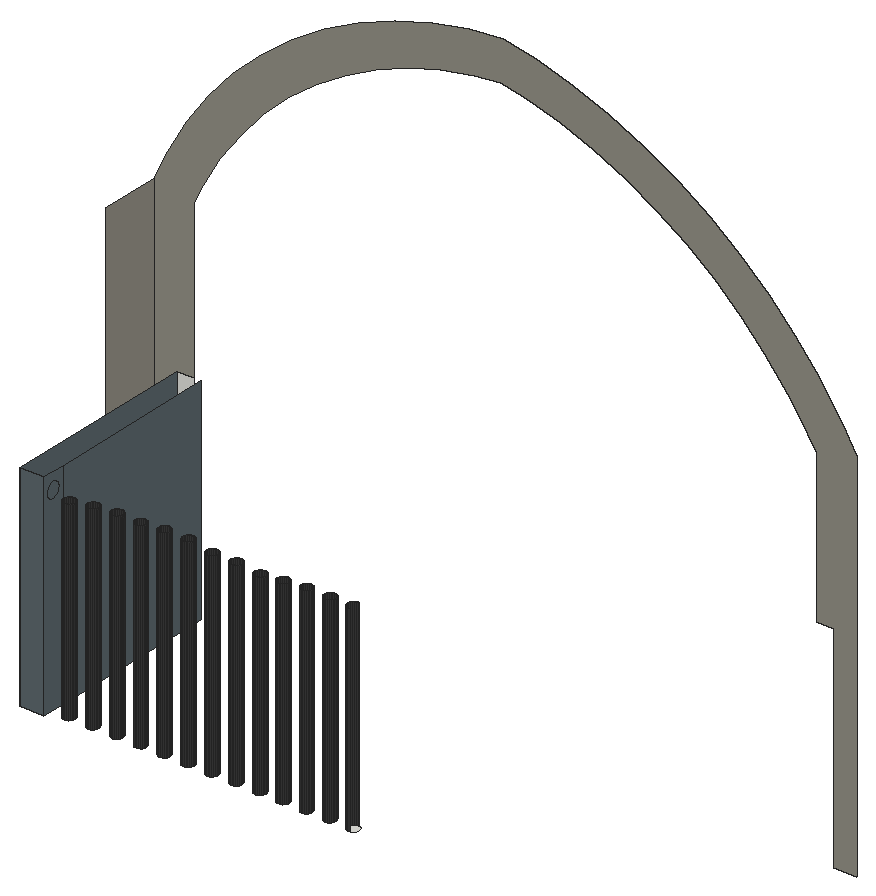
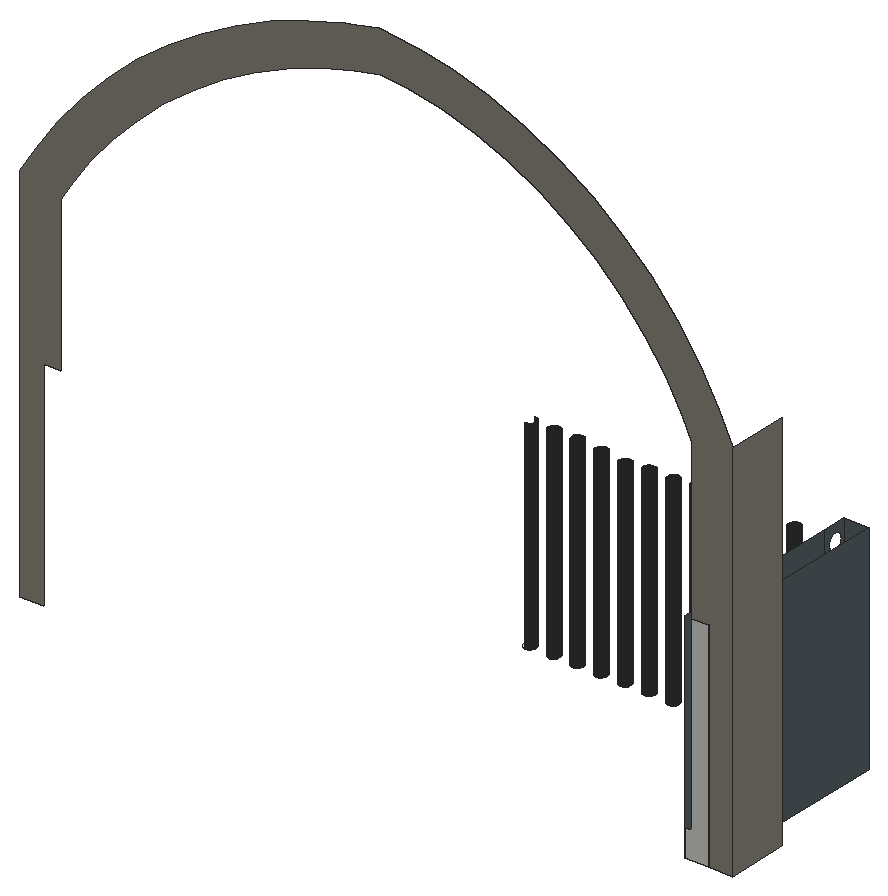
# SketchUp Ruby script. Lengths in inches.
U = 1.inch
M = Sketchup.active_model
def pt(a) = Geom::Point3d.new(a.map { |v| v * U })
def face(e, loops, mat)
  f = e.add_face(loops[0].map { |a| pt(a) })
  loops[1..].each { |l| e.add_face(l.map { |a| pt(a) }).erase! }
  f.material = f.back_material = mat if mat
  f
end
# faces: each face lists its corners as indices into pts; further lists are holes
def faces(e, pts, list, mat = nil) = list.each { |f| face(e, (f[0].is_a?(Array) ? f : [f]).map { |l| l.map { |i| pts[i] } }, mat) }
# xy, xz, yz: faces in a plane at the given z, y or x. An outline is a flat list of corners, or four numbers for a rectangle; further outlines are holes
def ring(l) = l.size == 4 ? [[l[0], l[1]], [l[2], l[1]], [l[2], l[3]], [l[0], l[3]]] : l.each_slice(2).to_a
def flat(e, list, mat, &to3) = list.each { |f| face(e, (f[0].is_a?(Array) ? f : [f]).map { |l| ring(l).map { |u, v| to3.(u, v) } }, mat) }
def xy(e, z, list, mat = nil) = flat(e, list, mat) { |x, y| [x, y, z] }
def xz(e, y, list, mat = nil) = flat(e, list, mat) { |x, z| [x, y, z] }
def yz(e, x, list, mat = nil) = flat(e, list, mat) { |y, z| [x, y, z] }
def lines(e, pts, list) = list.each { |a, b| e.add_line(pt(pts[a]), pt(pts[b])) }
# prism: a flat outline (further loops are holes) pulled along v
def prism(e, loops, v, mat = nil)
  f = face(e, loops, mat); d = Geom::Vector3d.new(v.map { |x| x * U })
  f.pushpull(f.normal.samedirection?(d) ? d.length : -d.length)
end
def box(e, o, s, mat = nil) = prism(e, [[o, [o[0] + s[0], o[1], o[2]], [o[0] + s[0], o[1] + s[1], o[2]], [o[0], o[1] + s[1], o[2]]]], [0, 0, s[2]], mat)
def at(x, y, z, deg = 0) = Geom::Transformation.translation(pt([x, y, z])) * Geom::Transformation.rotation(ORIGIN, Z_AXIS, deg.degrees)
def axes(o, x, y, z) = Geom::Transformation.new([*x, 0, *y, 0, *z, 0, *pt(o).to_a, 1])
def part(name) = M.definitions.add(name)
# library, detail: a bought-in or finely detailed component or shape, given as its bounding box
def library(name, o, s) = part(name).tap { |d| box(d.entities, o, s) }
def detail(e, o, s) = box(e.add_group.entities, o, s)
def put(e, d, t, mat = nil) = e.add_instance(d, t).tap { |i| i.material = mat if mat }
def group(e, t, mat = nil) = e.add_group.tap { |g| g.transformation = t; g.material = mat if mat }.entities
root = M.entities
M.materials.add("[Color M07]").color = [58, 58, 58]
M.materials.add("[Formica Graystone]").color = [149, 146, 135]
M.materials.add("[Formica Speckled Grey]").color = [94, 105, 111]
xy(root,334.79,[[221.4,120.91,224.22,144.04],[226.04,121.51,225.87,121.56,225.71,121.65,225.59,121.78,225.5,121.93,225.46,122.11,225.46,122.28,225.51,122.46,225.6,122.61,225.73,122.74,225.88,122.83,226.06,122.87,226.23,122.87,226.41,122.82,226.5625,122.73,226.6875,122.6,226.78,122.45,226.82,122.27,226.82,122.09,226.77,121.92,226.68,121.76,226.55,121.64,226.4,121.55,226.22,121.51],[228.85,121.51,228.68,121.56,228.53,121.65,228.4,121.78,228.3125,121.93,228.27,122.11,228.27,122.28,228.32,122.46,228.41,122.61,228.54,122.74,228.69,122.83,228.87,122.87,229.05,122.87,229.22,122.82,229.375,122.73,229.5,122.6,229.59,122.45,229.63,122.27,229.63,122.09,229.58,121.92,229.49,121.76,229.36,121.64,229.21,121.55,229.03,121.51],[231.67,121.51,231.49,121.56,231.34,121.65,231.21,121.78,231.125,121.93,231.08,122.11,231.08,122.28,231.13,122.46,231.22,122.61,231.35,122.74,231.51,122.83,231.68,122.87,231.86,122.87,232.03,122.82,232.1875,122.73,232.3125,122.6,232.4,122.45,232.45,122.27,232.44,122.09,232.4,121.92,232.3,121.76,232.18,121.64,232.02,121.55,231.85,121.51],[234.48,121.51,234.31,121.56,234.15,121.65,234.03,121.78,233.9375,121.93,233.89,122.11,233.9,122.28,233.94,122.46,234.03,122.61,234.16,122.74,234.32,122.83,234.49,122.87,234.67,122.87,234.85,122.82,235,122.73,235.125,122.6,235.21,122.45,235.26,122.27,235.26,122.09,235.21,121.92,235.12,121.76,234.99,121.64,234.83,121.55,234.66,121.51],
  [237.29,121.51,237.12,121.56,236.96,121.65,236.84,121.78,236.75,121.93,236.71,122.11,236.71,122.28,236.76,122.46,236.85,122.61,236.98,122.74,237.13,122.83,237.31,122.87,237.48,122.87,237.66,122.82,237.8125,122.73,237.9375,122.6,238.03,122.45,238.07,122.27,238.07,122.09,238.02,121.92,237.93,121.76,237.8,121.64,237.65,121.55,237.47,121.51],[240.1,121.51,239.93,121.56,239.78,121.65,239.65,121.78,239.5625,121.93,239.52,122.11,239.52,122.28,239.57,122.46,239.66,122.61,239.79,122.74,239.94,122.83,240.12,122.87,240.3,122.87,240.47,122.82,240.625,122.73,240.75,122.6,240.84,122.45,240.88,122.27,240.88,122.09,240.83,121.92,240.74,121.76,240.61,121.64,240.46,121.55,240.28,121.51],[242.92,121.51,242.74,121.56,242.59,121.65,242.46,121.78,242.375,121.93,242.33,122.11,242.33,122.28,242.38,122.46,242.47,122.61,242.6,122.74,242.76,122.83,242.93,122.87,243.11,122.87,243.28,122.82,243.4375,122.73,243.5625,122.6,243.65,122.45,243.7,122.27,243.69,122.09,243.65,121.92,243.55,121.76,243.43,121.64,243.27,121.55,243.1,121.51],[245.73,121.51,245.56,121.56,245.4,121.65,245.28,121.78,245.1875,121.93,245.14,122.11,245.15,122.28,245.19,122.46,245.28,122.61,245.41,122.74,245.57,122.83,245.74,122.87,245.92,122.87,246.1,122.82,246.25,122.73,246.375,122.6,246.46,122.45,246.51,122.27,246.51,122.09,246.46,121.92,246.37,121.76,246.24,121.64,246.08,121.55,245.91,121.51],[248.54,121.51,248.37,121.56,248.21,121.65,248.09,121.78,248,121.93,247.96,122.11,247.96,122.28,248.01,122.46,248.1,122.61,248.23,122.74,248.38,122.83,248.56,122.87,248.73,122.87,248.91,122.82,249.0625,122.73,249.1875,122.6,249.28,122.45,249.32,122.27,249.32,122.09,249.27,121.92,249.18,121.76,249.05,121.64,248.9,121.55,248.72,121.51],
  [251.29,121.51,251.12,121.56,250.96,121.65,250.84,121.78,250.75,121.93,250.71,122.11,250.71,122.28,250.76,122.46,250.85,122.61,250.98,122.74,251.13,122.83,251.31,122.87,251.48,122.87,251.66,122.82,251.8125,122.73,251.9375,122.6,252.03,122.45,252.07,122.27,252.07,122.09,252.02,121.92,251.93,121.76,251.8,121.64,251.65,121.55,251.47,121.51],[254.04,121.51,253.87,121.56,253.71,121.65,253.59,121.78,253.5,121.93,253.46,122.11,253.46,122.28,253.51,122.46,253.6,122.61,253.73,122.74,253.88,122.83,254.06,122.87,254.23,122.87,254.41,122.82,254.5625,122.73,254.6875,122.6,254.78,122.45,254.82,122.27,254.82,122.09,254.77,121.92,254.68,121.76,254.55,121.64,254.4,121.55,254.22,121.51],[256.79,121.51,256.62,121.56,256.46,121.65,256.34,121.78,256.25,121.93,256.21,122.11,256.21,122.28,256.26,122.46,256.35,122.61,256.48,122.74,256.63,122.83,256.81,122.87,256.98,122.87,257.16,122.82,257.3125,122.73,257.4375,122.6,257.53,122.45,257.57,122.27,257.57,122.09,257.52,121.92,257.43,121.76,257.3,121.64,257.15,121.55,256.97,121.51],[259.54,121.51,259.37,121.56,259.21,121.65,259.09,121.78,259,121.93,258.96,122.11,258.96,122.28,259.01,122.46,259.1,122.61,259.23,122.74,259.38,122.83,259.56,122.87,259.73,122.87,259.91,122.82,260.0625,122.73,260.1875,122.6,260.28,122.45,260.32,122.27,260.32,122.09,260.27,121.92,260.18,121.76,260.05,121.64,259.9,121.55,259.72,121.51]])
xz(root,120.91,[[221.4,334.79,224.22,359.98]],"[Formica Speckled Grey]")
xz(root,121.51,[[226.04,334.79,226.22,357.6],[228.85,334.79,229.03,358.07],[231.67,334.79,231.85,358.31],[234.48,334.79,234.66,358.31],[237.29,334.79,237.47,358.53],
  [240.1,334.79,240.28,358.53],[242.92,334.79,243.1,358.07],[245.73,334.79,245.91,358.07],[248.54,334.79,248.72,357.79],[251.29,334.79,251.47,358.07],
  [254.04,334.79,254.22,358.31],[256.79,334.79,256.97,358.31],[259.54,334.79,259.72,358.31]],"[Color M07]")
xz(root,122.87,[[226.06,334.79,226.23,357.6],[228.87,334.79,229.05,358.07],[231.68,334.79,231.86,358.31],[234.49,334.79,234.67,358.31],[237.31,334.79,237.48,358.53],
  [240.12,334.79,240.3,358.53],[242.93,334.79,243.11,358.07],[245.74,334.79,245.92,358.07],[248.56,334.79,248.73,357.79],[251.31,334.79,251.48,358.07],
  [254.06,334.79,254.23,358.31],[256.81,334.79,256.98,358.31],[259.56,334.79,259.73,358.31]],"[Color M07]")
xz(root,144.04,[[221.4,334.79,224.22,334.79,224.22,337.93,223.375,337.93,223.375,359.98,221.4,359.98]])
xz(root,144.04,[[218.68,334.79,221.4,334.79,221.4,359.98,223.375,359.98,223.375,378.37,224.41,380.625,226.46,384.17,228.84,387.5,231.52,390.6,234.47,393.42,237.6875,395.96,241.125,398.18,244.76,400.07,248.55,401.61,252.47,402.78,256.49,403.57,259.55,403.88,262.55,403.25,266.5625,402.09,270.47,400.625,274.27,398.875,277.91,396.84,281.4,394.54,284.7,391.99,287.8,389.1875,290.6875,386.17,293.33,382.9375,295.73,379.52,296.73,377.84,296.73,359.98,298.73,359.98,298.73,334.79,301.43,334.79,301.43,379.13,299.68,382.07,297.08,385.78,294.21,389.28,291.08,392.56,287.72,395.59,284.14,398.37,280.36,400.86,276.4,403.07,272.29,404.97,268.04,406.55,263.69,407.82,262.44,408.08,259.8,408.63,255.79,408.23,255.1,408.09,251.34,407.34,246.99,406.05,242.79,404.34,238.76,402.25,234.95,399.79,231.39,396.98,228.11,393.84,225.14,390.41,222.51,386.72,220.23,382.79,218.68,379.39]],"[Formica Graystone]")
yz(root,218.68,[[136.91,334.79,144.04,379.39]],"[Formica Graystone]")
yz(root,221.4,[[120.91,334.79,144.04,359.98]],"[Formica Speckled Grey]")
yz(root,224.22,[[[120.91,334.79,123.73,359.98],[122.22,357.13,121.97,357.16,121.75,357.25,121.55,357.4,121.41,357.6,121.3125,357.82,121.28,358.07,121.3125,358.31,121.41,358.53,121.55,358.73,121.75,358.88,121.97,358.97,122.22,359,122.46,358.97,122.6875,358.88,122.88,358.73,123.03,358.53,123.125,358.31,123.16,358.07,123.125,357.82,123.03,357.6,122.88,357.4,122.6875,357.25,122.46,357.16]],[123.73,334.79,144.04,359.98]],"[Formica Speckled Grey]")
yz(root,225.46,[[122.11,334.79,122.28,357.6]],"[Color M07]")
yz(root,226.82,[[122.09,334.79,122.27,357.6]],"[Color M07]")
yz(root,228.27,[[122.11,334.79,122.28,358.07]],"[Color M07]")
yz(root,229.63,[[122.09,334.79,122.27,358.07]],"[Color M07]")
yz(root,231.08,[[122.11,334.79,122.28,358.31]],"[Color M07]")
yz(root,235.26,[[122.09,334.79,122.27,358.31]],"[Color M07]")
yz(root,236.71,[[122.11,334.79,122.28,358.53]],"[Color M07]")
yz(root,238.07,[[122.09,334.79,122.27,358.53]],"[Color M07]")
yz(root,239.52,[[122.11,334.79,122.28,358.53]],"[Color M07]")
yz(root,240.88,[[122.09,334.79,122.27,358.53]],"[Color M07]")
yz(root,242.33,[[122.11,334.79,122.28,358.07]],"[Color M07]")
yz(root,246.51,[[122.09,334.79,122.27,358.07]],"[Color M07]")
yz(root,247.96,[[122.11,334.79,122.28,357.79]],"[Color M07]")
yz(root,249.32,[[122.09,334.79,122.27,357.79]],"[Color M07]")
yz(root,250.71,[[122.11,334.79,122.28,358.07]],"[Color M07]")
yz(root,252.07,[[122.09,334.79,122.27,358.07]],"[Color M07]")
yz(root,253.46,[[122.11,334.79,122.28,358.31]],"[Color M07]")
yz(root,254.82,[[122.09,334.79,122.27,358.31]],"[Color M07]")
yz(root,256.21,[[122.11,334.79,122.28,358.31]],"[Color M07]")
yz(root,257.57,[[122.09,334.79,122.27,358.31]],"[Color M07]")
yz(root,258.96,[[122.11,334.79,122.28,358.31]],"[Color M07]")
p = [[225.87,121.56,334.79],[226.04,121.51,334.79],[226.04,121.51,357.6],[225.87,121.56,357.6],[225.87,121.56,357.4],[226.22,121.51,334.79],
  [226.4,121.55,334.79],[226.4,121.55,357.6],[226.22,121.51,357.6],[228.68,121.56,334.79],[228.85,121.51,334.79],[228.85,121.51,358.07],
  [228.68,121.56,358.07],[228.68,121.56,357.4],[229.03,121.51,334.79],[229.21,121.55,334.79],[229.21,121.55,358.07],[229.03,121.51,358.07],
  [231.49,121.56,334.79],[231.67,121.51,334.79],[231.67,121.51,358.31],[231.49,121.56,358.31],[231.49,121.56,357.4],[231.85,121.51,334.79],
  [232.02,121.55,334.79],[232.02,121.55,358.31],[231.85,121.51,358.31],[234.31,121.56,334.79],[234.48,121.51,334.79],[234.48,121.51,358.31],
  [234.31,121.56,358.31],[234.31,121.56,357.4],[234.66,121.51,334.79],[234.83,121.55,334.79],[234.83,121.55,358.31],[234.66,121.51,358.31],
  [237.12,121.56,334.79],[237.29,121.51,334.79],[237.29,121.51,358.53],[237.12,121.56,358.53],[237.12,121.56,357.4],[237.47,121.51,334.79],
  [237.65,121.55,334.79],[237.65,121.55,358.53],[237.47,121.51,358.53],[239.93,121.56,334.79],[240.1,121.51,334.79],[240.1,121.51,358.53],
  [239.93,121.56,358.53],[239.93,121.56,357.4],[240.28,121.51,334.79],[240.46,121.55,334.79],[240.46,121.55,358.53],[240.28,121.51,358.53],
  [242.74,121.56,334.79],[242.92,121.51,334.79],[242.92,121.51,358.07],[242.74,121.56,358.07],[242.74,121.56,357.4],[243.1,121.51,334.79],
  [243.27,121.55,334.79],[243.27,121.55,358.07],[243.1,121.51,358.07],[245.56,121.56,334.79],[245.73,121.51,334.79],[245.73,121.51,358.07],
  [245.56,121.56,358.07],[245.56,121.56,357.4],[245.91,121.51,334.79],[246.08,121.55,334.79],[246.08,121.55,358.07],[245.91,121.51,358.07],
  [248.37,121.56,334.79],[248.54,121.51,334.79],[248.54,121.51,357.79],[248.37,121.56,357.79],[248.37,121.56,357.4],[248.72,121.51,334.79],
  [248.9,121.55,334.79],[248.9,121.55,357.79],[248.72,121.51,357.79],[251.12,121.56,334.79],[251.29,121.51,334.79],[251.29,121.51,358.07],
  [251.12,121.56,358.07],[251.12,121.56,357.4],[251.47,121.51,334.79],[251.65,121.55,334.79],[251.65,121.55,358.07],[251.47,121.51,358.07],
  [253.87,121.56,334.79],[254.04,121.51,334.79],[254.04,121.51,358.31],[253.87,121.56,358.31],[253.87,121.56,357.4],[254.22,121.51,334.79],
  [254.4,121.55,334.79],[254.4,121.55,358.31],[254.22,121.51,358.31],[256.62,121.56,334.79],[256.79,121.51,334.79],[256.79,121.51,358.31],
  [256.62,121.56,358.31],[256.62,121.56,357.4],[256.97,121.51,334.79],[257.15,121.55,334.79],[257.15,121.55,358.31],[256.97,121.51,358.31],
  [259.37,121.56,334.79],[259.54,121.51,334.79],[259.54,121.51,358.31],[259.37,121.56,358.31],[259.37,121.56,357.4],[225.59,121.78,334.79],
  [225.71,121.65,334.79],[225.71,121.65,357.6],[225.59,121.78,357.6],[226.55,121.64,334.79],[226.55,121.64,357.6],[226.68,121.76,334.79],
  [226.68,121.76,357.6],[228.4,121.78,334.79],[228.53,121.65,334.79],[228.53,121.65,358.07],[228.4,121.78,358.07],[229.36,121.64,334.79],
  [229.36,121.64,358.07],[229.49,121.76,334.79],[229.49,121.76,358.07],[231.21,121.78,334.79],[231.34,121.65,334.79],[231.34,121.65,358.31],
  [231.21,121.78,358.31],[232.18,121.64,334.79],[232.18,121.64,358.31],[232.3,121.76,334.79],[232.3,121.76,358.31],[234.03,121.78,334.79],
  [234.15,121.65,334.79],[234.15,121.65,358.31],[234.03,121.78,358.31],[234.99,121.64,334.79],[234.99,121.64,358.31],[235.12,121.76,334.79],
  [235.12,121.76,358.31],[236.84,121.78,334.79],[236.96,121.65,334.79],[236.96,121.65,358.53],[236.84,121.78,358.53],[237.8,121.64,334.79],
  [237.8,121.64,358.53],[237.93,121.76,334.79],[237.93,121.76,358.53],[239.65,121.78,334.79],[239.78,121.65,334.79],[239.78,121.65,358.53],
  [239.65,121.78,358.53],[240.61,121.64,334.79],[240.61,121.64,358.53],[240.74,121.76,334.79],[240.74,121.76,358.53],[242.46,121.78,334.79],
  [242.59,121.65,334.79],[242.59,121.65,358.07],[242.46,121.78,358.07],[243.43,121.64,334.79],[243.43,121.64,358.07],[243.55,121.76,334.79],
  [243.55,121.76,358.07],[245.28,121.78,334.79],[245.4,121.65,334.79],[245.4,121.65,358.07],[245.28,121.78,358.07],[246.24,121.64,334.79],
  [246.24,121.64,358.07],[246.37,121.76,334.79],[246.37,121.76,358.07],[248.09,121.78,334.79],[248.21,121.65,334.79],[248.21,121.65,357.79],
  [248.09,121.78,357.79],[249.05,121.64,334.79],[249.05,121.64,357.79],[249.18,121.76,334.79],[249.18,121.76,357.79],[250.84,121.78,334.79],
  [250.96,121.65,334.79],[250.96,121.65,358.07],[250.84,121.78,358.07],[251.8,121.64,334.79],[251.8,121.64,358.07],[251.93,121.76,334.79],
  [251.93,121.76,358.07],[253.59,121.78,334.79],[253.71,121.65,334.79],[253.71,121.65,358.31],[253.59,121.78,358.31],[254.55,121.64,334.79],
  [254.55,121.64,358.31],[254.68,121.76,334.79],[254.68,121.76,358.31],[256.34,121.78,334.79],[256.46,121.65,334.79],[256.46,121.65,358.31],
  [256.34,121.78,358.31],[257.3,121.64,334.79],[257.3,121.64,358.31],[257.43,121.76,334.79],[257.43,121.76,358.31],[259.09,121.78,334.79],
  [259.21,121.65,334.79],[259.21,121.65,358.31],[259.09,121.78,358.31],[225.5,121.93,334.79],[225.5,121.93,357.6],[226.77,121.92,334.79],
  [226.77,121.92,357.6],[228.3125,121.93,334.79],[228.3125,121.93,358.07],[229.58,121.92,334.79],[229.58,121.92,358.07],[231.125,121.93,334.79],
  [231.125,121.93,358.31],[232.4,121.92,334.79],[232.4,121.92,358.31],[233.9375,121.93,334.79],[233.9375,121.93,358.31],[235.21,121.92,334.79],
  [235.21,121.92,358.31],[236.75,121.93,334.79],[236.75,121.93,358.53],[238.02,121.92,334.79],[238.02,121.92,358.53],[239.5625,121.93,334.79],
  [239.5625,121.93,358.53],[240.83,121.92,334.79],[240.83,121.92,358.53],[242.375,121.93,334.79],[242.375,121.93,358.07],[243.65,121.92,334.79],
  [243.65,121.92,358.07],[245.1875,121.93,334.79],[245.1875,121.93,358.07],[246.46,121.92,334.79],[246.46,121.92,358.07],[248,121.93,334.79],
  [248,121.93,357.79],[249.27,121.92,334.79],[249.27,121.92,357.79],[250.75,121.93,334.79],[250.75,121.93,358.07],[252.02,121.92,334.79],
  [252.02,121.92,358.07],[253.5,121.93,334.79],[253.5,121.93,358.31],[254.77,121.92,334.79],[254.77,121.92,358.31],[256.25,121.93,334.79],
  [256.25,121.93,358.31],[257.52,121.92,334.79],[257.52,121.92,358.31],[259,121.93,334.79],[259,121.93,358.31],[225.46,122.11,334.79],
  [225.46,122.11,357.6],[226.82,122.09,334.79],[226.82,122.09,357.6],[228.27,122.11,334.79],[228.27,122.11,358.07],[229.63,122.09,334.79],
  [229.63,122.09,358.07],[231.08,122.11,334.79],[231.08,122.11,358.31],[232.44,122.09,334.79],[232.44,122.09,358.31],[233.89,122.11,334.79],
  [233.89,122.11,358.31],[235.26,122.09,334.79],[235.26,122.09,358.31],[236.71,122.11,334.79],[236.71,122.11,358.53],[238.07,122.09,334.79],
  [238.07,122.09,358.53],[239.52,122.11,334.79],[239.52,122.11,358.53],[240.88,122.09,334.79],[240.88,122.09,358.53],[242.33,122.11,334.79],
  [242.33,122.11,358.07],[243.69,122.09,334.79],[243.69,122.09,358.07],[245.14,122.11,334.79],[245.14,122.11,358.07],[246.51,122.09,334.79],
  [246.51,122.09,358.07],[247.96,122.11,334.79],[247.96,122.11,357.79],[249.32,122.09,334.79],[249.32,122.09,357.79],[250.71,122.11,334.79],
  [250.71,122.11,358.07],[252.07,122.09,334.79],[252.07,122.09,358.07],[253.46,122.11,334.79],[253.46,122.11,358.31],[254.82,122.09,334.79],
  [254.82,122.09,358.31],[256.21,122.11,334.79],[256.21,122.11,358.31],[257.57,122.09,334.79],[257.57,122.09,358.31],[258.96,122.11,334.79],
  [258.96,122.11,358.31],[232.45,122.27,334.79],[232.45,122.27,358.31],[233.9,122.28,334.79],[233.9,122.28,358.31],[243.7,122.27,334.79],
  [243.7,122.27,358.07],[245.15,122.28,334.79],[245.15,122.28,358.07],[225.51,122.46,334.79],[225.46,122.28,334.79],[225.46,122.28,357.6],
  [225.51,122.46,357.6],[226.82,122.27,334.79],[226.78,122.45,334.79],[226.78,122.45,357.6],[226.82,122.27,357.6],[228.32,122.46,334.79],
  [228.27,122.28,334.79],[228.27,122.28,358.07],[228.32,122.46,358.07],[229.63,122.27,334.79],[229.59,122.45,334.79],[229.59,122.45,358.07],
  [229.63,122.27,358.07],[231.13,122.46,334.79],[231.08,122.28,334.79],[231.08,122.28,358.31],[231.13,122.46,358.31],[232.4,122.45,334.79],
  [232.4,122.45,358.31],[233.94,122.46,334.79],[233.94,122.46,358.31],[235.26,122.27,334.79],[235.21,122.45,334.79],[235.21,122.45,358.31],
  [235.26,122.27,358.31],[236.76,122.46,334.79],[236.71,122.28,334.79],[236.71,122.28,358.53],[236.76,122.46,358.53],[238.07,122.27,334.79],
  [238.03,122.45,334.79],[238.03,122.45,358.53],[238.07,122.27,358.53],[239.57,122.46,334.79],[239.52,122.28,334.79],[239.52,122.28,358.53],
  [239.57,122.46,358.53],[240.88,122.27,334.79],[240.84,122.45,334.79],[240.84,122.45,358.53],[240.88,122.27,358.53],[242.38,122.46,334.79],
  [242.33,122.28,334.79],[242.33,122.28,358.07],[242.38,122.46,358.07],[243.65,122.45,334.79],[243.65,122.45,358.07],[245.19,122.46,334.79],
  [245.19,122.46,358.07],[246.51,122.27,334.79],[246.46,122.45,334.79],[246.46,122.45,358.07],[246.51,122.27,358.07],[248.01,122.46,334.79],
  [247.96,122.28,334.79],[247.96,122.28,357.79],[248.01,122.46,357.79],[249.32,122.27,334.79],[249.28,122.45,334.79],[249.28,122.45,357.79],
  [249.32,122.27,357.79],[250.76,122.46,334.79],[250.71,122.28,334.79],[250.71,122.28,358.07],[250.76,122.46,358.07],[252.07,122.27,334.79],
  [252.03,122.45,334.79],[252.03,122.45,358.07],[252.07,122.27,358.07],[253.51,122.46,334.79],[253.46,122.28,334.79],[253.46,122.28,358.31],
  [253.51,122.46,358.31],[254.82,122.27,334.79],[254.78,122.45,334.79],[254.78,122.45,358.31],[254.82,122.27,358.31],[256.26,122.46,334.79],
  [256.21,122.28,334.79],[256.21,122.28,358.31],[256.26,122.46,358.31],[257.57,122.27,334.79],[257.53,122.45,334.79],[257.53,122.45,358.31],
  [257.57,122.27,358.31],[259.01,122.46,334.79],[258.96,122.28,334.79],[258.96,122.28,358.31],[259.01,122.46,358.31],[226.6875,122.6,334.79],
  [226.6875,122.6,357.6],[229.5,122.6,334.79],[229.5,122.6,358.07],[232.3125,122.6,334.79],[232.3125,122.6,358.31],[235.125,122.6,334.79],
  [235.125,122.6,358.31],[237.9375,122.6,334.79],[237.9375,122.6,358.53],[240.75,122.6,334.79],[240.75,122.6,358.53],[243.5625,122.6,334.79],
  [243.5625,122.6,358.07],[246.375,122.6,334.79],[246.375,122.6,358.07],[249.1875,122.6,334.79],[249.1875,122.6,357.79],[251.9375,122.6,334.79],
  [251.9375,122.6,358.07],[254.6875,122.6,334.79],[254.6875,122.6,358.31],[257.4375,122.6,334.79],[257.4375,122.6,358.31],[225.6,122.61,334.79],
  [225.6,122.61,357.6],[228.41,122.61,334.79],[228.41,122.61,358.07],[231.22,122.61,334.79],[231.22,122.61,358.31],[234.03,122.61,334.79],
  [234.03,122.61,358.31],[236.85,122.61,334.79],[236.85,122.61,358.53],[239.66,122.61,334.79],[239.66,122.61,358.53],[242.47,122.61,334.79],
  [242.47,122.61,358.07],[245.28,122.61,334.79],[245.28,122.61,358.07],[248.1,122.61,334.79],[248.1,122.61,357.79],[250.85,122.61,334.79],
  [250.85,122.61,358.07],[253.6,122.61,334.79],[253.6,122.61,358.31],[256.35,122.61,334.79],[256.35,122.61,358.31],[259.1,122.61,334.79],
  [259.1,122.61,358.31],[225.73,122.74,334.79],[225.73,122.74,357.6],[226.5625,122.73,334.79],[226.5625,122.73,357.6],[228.54,122.74,334.79],
  [228.54,122.74,358.07],[229.375,122.73,334.79],[229.375,122.73,358.07],[231.35,122.74,334.79],[231.35,122.74,358.31],[232.1875,122.73,334.79],
  [232.1875,122.73,358.31],[234.16,122.74,334.79],[234.16,122.74,358.31],[235,122.73,334.79],[235,122.73,358.31],[236.98,122.74,334.79],
  [236.98,122.74,358.53],[237.8125,122.73,334.79],[237.8125,122.73,358.53],[239.79,122.74,334.79],[239.79,122.74,358.53],[240.625,122.73,334.79],
  [240.625,122.73,358.53],[242.6,122.74,334.79],[242.6,122.74,358.07],[243.4375,122.73,334.79],[243.4375,122.73,358.07],[245.41,122.74,334.79],
  [245.41,122.74,358.07],[246.25,122.73,334.79],[246.25,122.73,358.07],[248.23,122.74,334.79],[248.23,122.74,357.79],[249.0625,122.73,334.79],
  [249.0625,122.73,357.79],[250.98,122.74,334.79],[250.98,122.74,358.07],[251.8125,122.73,334.79],[251.8125,122.73,358.07],[253.73,122.74,334.79],
  [253.73,122.74,358.31],[254.5625,122.73,334.79],[254.5625,122.73,358.31],[256.48,122.74,334.79],[256.48,122.74,358.31],[257.3125,122.73,334.79],
  [257.3125,122.73,358.31],[259.23,122.74,334.79],[259.23,122.74,358.31],[225.88,122.83,334.79],[225.88,122.83,357.6],[226.41,122.82,334.79],
  [226.41,122.82,357.6],[228.69,122.83,334.79],[228.69,122.83,358.07],[229.22,122.82,334.79],[229.22,122.82,358.07],[231.51,122.83,334.79],
  [231.51,122.83,358.31],[232.03,122.82,334.79],[232.03,122.82,358.31],[234.32,122.83,334.79],[234.32,122.83,358.31],[234.85,122.82,334.79],
  [234.85,122.82,358.31],[237.13,122.83,334.79],[237.13,122.83,358.53],[237.66,122.82,334.79],[237.66,122.82,358.53],[239.94,122.83,334.79],
  [239.94,122.83,358.53],[240.47,122.82,334.79],[240.47,122.82,358.53],[242.76,122.83,334.79],[242.76,122.83,358.07],[243.28,122.82,334.79],
  [243.28,122.82,358.07],[245.57,122.83,334.79],[245.57,122.83,358.07],[246.1,122.82,334.79],[246.1,122.82,358.07],[248.38,122.83,334.79],
  [248.38,122.83,357.79],[248.91,122.82,334.79],[248.91,122.82,357.79],[251.13,122.83,334.79],[251.13,122.83,358.07],[251.66,122.82,334.79],
  [251.66,122.82,358.07],[253.88,122.83,334.79],[253.88,122.83,358.31],[254.41,122.82,334.79],[254.41,122.82,358.31],[256.63,122.83,334.79],
  [256.63,122.83,358.31],[257.16,122.82,334.79],[257.16,122.82,358.31],[259.38,122.83,334.79],[259.38,122.83,358.31],[226.06,122.87,334.79],
  [226.06,122.87,357.6],[226.23,122.87,334.79],[226.23,122.87,357.6],[228.87,122.87,334.79],[228.87,122.87,358.07],[229.05,122.87,334.79],
  [229.05,122.87,358.07],[231.68,122.87,334.79],[231.68,122.87,358.31],[231.86,122.87,334.79],[231.86,122.87,358.31],[234.49,122.87,334.79],
  [234.49,122.87,358.31],[234.67,122.87,334.79],[234.67,122.87,358.31],[237.31,122.87,334.79],[237.31,122.87,358.53],[237.48,122.87,334.79],
  [237.48,122.87,358.53],[240.12,122.87,334.79],[240.12,122.87,358.53],[240.3,122.87,334.79],[240.3,122.87,358.53],[242.93,122.87,334.79],
  [242.93,122.87,358.07],[243.11,122.87,334.79],[243.11,122.87,358.07],[245.74,122.87,334.79],[245.74,122.87,358.07],[245.92,122.87,334.79],
  [245.92,122.87,358.07],[248.56,122.87,334.79],[248.56,122.87,357.79],[248.73,122.87,334.79],[248.73,122.87,357.79],[251.31,122.87,334.79],
  [251.31,122.87,358.07],[251.48,122.87,334.79],[251.48,122.87,358.07],[254.06,122.87,334.79],[254.06,122.87,358.31],[254.23,122.87,334.79],
  [254.23,122.87,358.31],[256.81,122.87,334.79],[256.81,122.87,358.31],[256.98,122.87,334.79],[256.98,122.87,358.31],[259.56,122.87,334.79],
  [259.56,122.87,358.31]]
faces(root,p,[[0,1,2,3,4],[5,6,7,8],[9,10,11,12,13],[14,15,16,17],[18,19,20,21,22],[23,24,25,26],[27,28,29,30,31],[32,33,34,35],
  [36,37,38,39,40],[41,42,43,44],[45,46,47,48,49],[50,51,52,53],[54,55,56,57,58],[59,60,61,62],[63,64,65,66,67],[68,69,70,71],
  [72,73,74,75,76],[77,78,79,80],[81,82,83,84,85],[86,87,88,89],[90,91,92,93,94],[95,96,97,98],[99,100,101,102,103],[104,105,106,107],
  [108,109,110,111,112],[113,114,115,116],[114,0,4,3,115],[6,117,118,7],[117,119,120,118],[121,122,123,124],[122,9,13,12,123],[15,125,126,16],
  [125,127,128,126],[129,130,131,132],[130,18,22,21,131],[24,133,134,25],[133,135,136,134],[137,138,139,140],[138,27,31,30,139],[33,141,142,34],
  [141,143,144,142],[145,146,147,148],[146,36,40,39,147],[42,149,150,43],[149,151,152,150],[153,154,155,156],[154,45,49,48,155],[51,157,158,52],
  [157,159,160,158],[161,162,163,164],[162,54,58,57,163],[60,165,166,61],[165,167,168,166],[169,170,171,172],[170,63,67,66,171],[69,173,174,70],
  [173,175,176,174],[177,178,179,180],[178,72,76,75,179],[78,181,182,79],[181,183,184,182],[185,186,187,188],[186,81,85,84,187],[87,189,190,88],
  [189,191,192,190],[193,194,195,196],[194,90,94,93,195],[96,197,198,97],[197,199,200,198],[201,202,203,204],[202,99,103,102,203],[105,205,206,106],
  [205,207,208,206],[209,210,211,212],[210,108,112,111,211],[213,113,116,214],[119,215,216,120],[217,121,124,218],[127,219,220,128],[221,129,132,222],
  [135,223,224,136],[225,137,140,226],[143,227,228,144],[229,145,148,230],[151,231,232,152],[233,153,156,234],[159,235,236,160],[237,161,164,238],
  [167,239,240,168],[241,169,172,242],[175,243,244,176],[245,177,180,246],[183,247,248,184],[249,185,188,250],[191,251,252,192],[253,193,196,254],
  [199,255,256,200],[257,201,204,258],[207,259,260,208],[261,209,212,262],[263,213,214,264],[215,265,266,216],[267,217,218,268],[219,269,270,220],
  [271,221,222,272],[223,273,274,224],[275,225,226,276],[227,277,278,228],[279,229,230,280],[231,281,282,232],[283,233,234,284],[235,285,286,236],
  [287,237,238,288],[239,289,290,240],[291,241,242,292],[243,293,294,244],[295,245,246,296],[247,297,298,248],[299,249,250,300],[251,301,302,252],
  [303,253,254,304],[255,305,306,256],[307,257,258,308],[259,309,310,260],[311,261,262,312],[273,313,314,274],[315,275,276,316],[289,317,318,290],
  [319,291,292,320],[321,322,323,324],[325,326,327,328],[329,330,331,332],[333,334,335,336],[337,338,339,340],[313,341,342,314],[343,315,316,344],
  [345,346,347,348],[349,350,351,352],[353,354,355,356],[357,358,359,360],[361,362,363,364],[365,366,367,368],[317,369,370,318],[371,319,320,372],
  [373,374,375,376],[377,378,379,380],[381,382,383,384],[385,386,387,388],[389,390,391,392],[393,394,395,396],[397,398,399,400],[401,402,403,404],
  [405,406,407,408],[409,410,411,412],[326,413,414,327],[334,415,416,335],[341,417,418,342],[346,419,420,347],[354,421,422,355],[362,423,424,363],
  [369,425,426,370],[374,427,428,375],[382,429,430,383],[390,431,432,391],[398,433,434,399],[406,435,436,407],[437,321,324,438],[439,329,332,440],
  [441,337,340,442],[443,343,344,444],[445,349,352,446],[447,357,360,448],[449,365,368,450],[451,371,372,452],[453,377,380,454],[455,385,388,456],
  [457,393,396,458],[459,401,404,460],[461,409,412,462],[463,437,438,464],[413,465,466,414],[467,439,440,468],[415,469,470,416],[471,441,442,472],
  [417,473,474,418],[475,443,444,476],[419,477,478,420],[479,445,446,480],[421,481,482,422],[483,447,448,484],[423,485,486,424],[487,449,450,488],
  [425,489,490,426],[491,451,452,492],[427,493,494,428],[495,453,454,496],[429,497,498,430],[499,455,456,500],[431,501,502,432],[503,457,458,504],
  [433,505,506,434],[507,459,460,508],[435,509,510,436],[511,461,462,512],[513,463,464,514],[465,515,516,466],[517,467,468,518],[469,519,520,470],
  [521,471,472,522],[473,523,524,474],[525,475,476,526],[477,527,528,478],[529,479,480,530],[481,531,532,482],[533,483,484,534],[485,535,536,486],
  [537,487,488,538],[489,539,540,490],[541,491,492,542],[493,543,544,494],[545,495,496,546],[497,547,548,498],[549,499,500,550],[501,551,552,502],
  [553,503,504,554],[505,555,556,506],[557,507,508,558],[509,559,560,510],[561,511,512,562],[563,513,514,564],[515,565,566,516],[567,517,518,568],
  [519,569,570,520],[571,521,522,572],[523,573,574,524],[575,525,526,576],[527,577,578,528],[579,529,530,580],[531,581,582,532],[583,533,534,584],
  [535,585,586,536],[587,537,538,588],[539,589,590,540],[591,541,542,592],[543,593,594,544],[595,545,546,596],[547,597,598,548],[599,549,550,600],
  [551,601,602,552],[603,553,554,604],[555,605,606,556],[607,557,558,608],[559,609,610,560],[611,561,562,612]],"[Color M07]")
